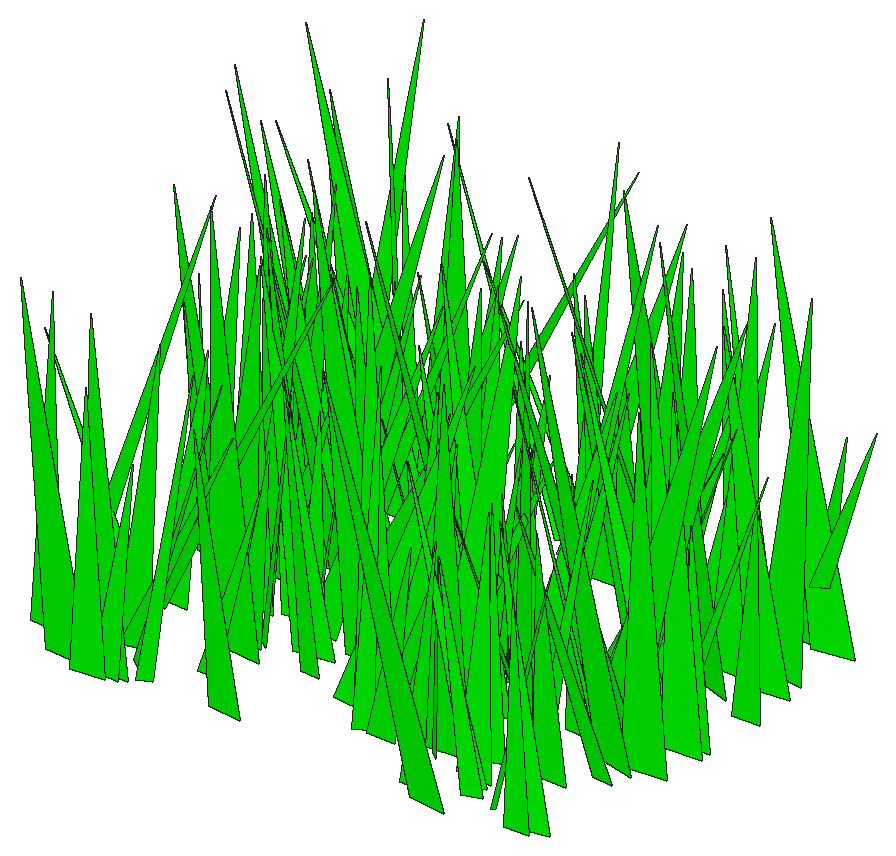
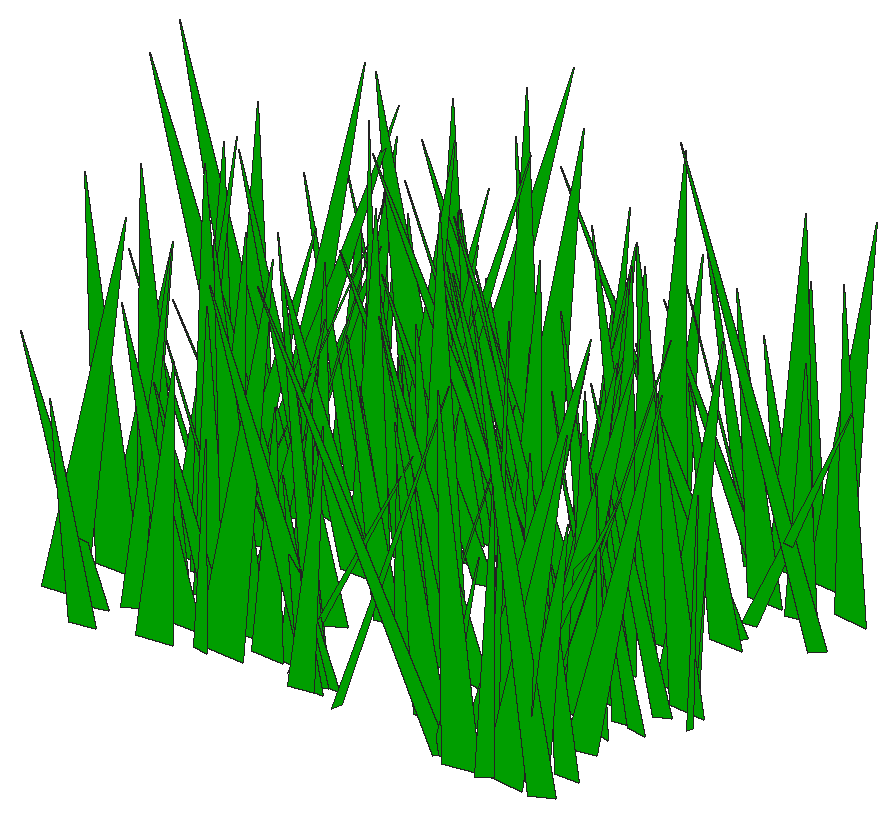
# SketchUp Ruby script. Lengths in inches.
U = 1.inch
M = Sketchup.active_model
def pt(a) = Geom::Point3d.new(a.map { |v| v * U })
def face(e, loops, mat)
  f = e.add_face(loops[0].map { |a| pt(a) })
  loops[1..].each { |l| e.add_face(l.map { |a| pt(a) }).erase! }
  f.material = f.back_material = mat if mat
  f
end
# faces: each face lists its corners as indices into pts; further lists are holes
def faces(e, pts, list, mat = nil) = list.each { |f| face(e, (f[0].is_a?(Array) ? f : [f]).map { |l| l.map { |i| pts[i] } }, mat) }
# xy, xz, yz: faces in a plane at the given z, y or x. An outline is a flat list of corners, or four numbers for a rectangle; further outlines are holes
def ring(l) = l.size == 4 ? [[l[0], l[1]], [l[2], l[1]], [l[2], l[3]], [l[0], l[3]]] : l.each_slice(2).to_a
def flat(e, list, mat, &to3) = list.each { |f| face(e, (f[0].is_a?(Array) ? f : [f]).map { |l| ring(l).map { |u, v| to3.(u, v) } }, mat) }
def xy(e, z, list, mat = nil) = flat(e, list, mat) { |x, y| [x, y, z] }
def xz(e, y, list, mat = nil) = flat(e, list, mat) { |x, z| [x, y, z] }
def yz(e, x, list, mat = nil) = flat(e, list, mat) { |y, z| [x, y, z] }
def lines(e, pts, list) = list.each { |a, b| e.add_line(pt(pts[a]), pt(pts[b])) }
# prism: a flat outline (further loops are holes) pulled along v
def prism(e, loops, v, mat = nil)
  f = face(e, loops, mat); d = Geom::Vector3d.new(v.map { |x| x * U })
  f.pushpull(f.normal.samedirection?(d) ? d.length : -d.length)
end
def box(e, o, s, mat = nil) = prism(e, [[o, [o[0] + s[0], o[1], o[2]], [o[0] + s[0], o[1] + s[1], o[2]], [o[0], o[1] + s[1], o[2]]]], [0, 0, s[2]], mat)
def at(x, y, z, deg = 0) = Geom::Transformation.translation(pt([x, y, z])) * Geom::Transformation.rotation(ORIGIN, Z_AXIS, deg.degrees)
def axes(o, x, y, z) = Geom::Transformation.new([*x, 0, *y, 0, *z, 0, *pt(o).to_a, 1])
def part(name) = M.definitions.add(name)
# library, detail: a bought-in or finely detailed component or shape, given as its bounding box
def library(name, o, s) = part(name).tap { |d| box(d.entities, o, s) }
def detail(e, o, s) = box(e.add_group.entities, o, s)
def put(e, d, t, mat = nil) = e.add_instance(d, t).tap { |i| i.material = mat if mat }
def group(e, t, mat = nil) = e.add_group.tap { |g| g.transformation = t; g.material = mat if mat }.entities
root = M.entities
M.materials.add("[0065_Lime]").color = [0, 255, 0]
c1 = part("fur_instance\#9")
p = [[0.8125,0,1.79],[0.67,-0.02,1.48],[0,-0.11,0],[0,0.11,0]]
faces(c1.entities,p,[[0,1,2,3]])
put(root,c1,axes([148.79,27.41,1.48],[-4.36413,0.0679,1.42951],[-0.40399,-0.66089,0.23585],[1.7773,0.0165,3.56374]),"[0065_Lime]")
put(root,c1,axes([150.34,30.25,1.48],[-6.51541,0.60637,1.27175],[-4.41577,-0.93218,-0.07461],[1.25175,-0.13226,6.35627]),"[0065_Lime]")
put(root,c1,axes([149.14,19.9,1.48],[3.62959,0.6982,2.01127],[-5.3272,0.55472,-0.09199],[-1.55669,-0.27041,5.00428]),"[0065_Lime]")
put(root,c1,axes([151.2,21.77,1.48],[-5.0487,0.24124,0.28222],[-1.73587,-0.70899,-0.23839],[0.23344,-0.05474,4.33106]),"[0065_Lime]")
put(root,c1,axes([150.35,32.46,1.48],[-2.61436,0.73575,0.51064],[-5.26778,-0.36894,-0.03169],[0.24537,-0.08138,4.76031]),"[0065_Lime]")
put(root,c1,axes([150.42,25.97,1.48],[-3.24186,-0.87839,1.38716],[6.44284,-0.46548,0.08559],[0.68891,0.21971,5.72721]),"[0065_Lime]")
put(root,c1,axes([152.13,32.04,1.48],[-6.23995,0.33949,0.21467],[-2.42526,-0.87643,-0.1994],[0.15736,-0.04553,5.43917]),"[0065_Lime]")
put(root,c1,axes([150.11,25.82,1.48],[-3.10048,-0.49021,1.16814],[3.63883,-0.45753,-0.04358],[0.99584,0.14559,3.79617]),"[0065_Lime]")
put(root,c1,axes([149.48,26.69,1.48],[2.5445,0.77902,1.23454],[-5.70579,0.37053,-0.05376],[-0.69495,-0.18982,4.96153]),"[0065_Lime]")
put(root,c1,axes([150.26,20.69,1.48],[-2.31714,0.67871,0.78015],[-4.863,-0.33882,0.32078],[0.77494,-0.09683,4.34572]),"[0065_Lime]")
put(root,c1,axes([150.95,32.95,1.48],[-3.51919,-0.90206,0.91897],[6.49484,-0.50053,-0.00735],[0.55111,0.13859,5.95488]),"[0065_Lime]")
put(root,c1,axes([150.71,18.86,1.48],[-2.47516,-0.99817,1.03588],[7.20412,-0.35294,-0.007],[0.42726,0.16858,6.11882]),"[0065_Lime]")
put(root,c1,axes([149.74,31.65,1.48],[2.54664,-0.49635,0.67652],[3.56798,0.36853,0.17373],[-0.66219,0.07682,3.53783]),"[0065_Lime]")
put(root,c1,axes([150.4,29.22,1.48],[4.29122,0.27494,1.64911],[-2.16036,0.65427,0.06434],[-1.80871,-0.12918,3.83571]),"[0065_Lime]")
put(root,c1,axes([150.35,28.31,1.48],[-0.84315,0.57058,1.0024],[-4.1932,-0.13912,0.31998],[0.65123,-0.15706,3.35818]),"[0065_Lime]")
put(root,c1,axes([152.72,28.54,1.48],[-8.21693,-0.01318,1.13181],[0.1147,-1.17091,0.0942],[1.38986,0.01873,6.68353]),"[0065_Lime]")
put(root,c1,axes([149.86,28.42,1.48],[4.47885,0.44067,1.13492],[-3.27298,0.6454,0.14884],[-1.03398,-0.13413,4.44494]),"[0065_Lime]")
put(root,c1,axes([149.6,32.9,1.48],[8.12572,-0.44878,2.16792],[3.45574,1.18577,-0.34466],[-2.31551,0.19477,7.09341]),"[0065_Lime]")
put(root,c1,axes([153.06,30.97,1.48],[-6.84359,0.82325,1.04818],[-5.93268,-0.96951,-0.11241],[0.888,-0.13265,7.32705]),"[0065_Lime]")
put(root,c1,axes([149.8,27.35,1.48],[5.49629,-0.3427,1.04891],[2.54858,0.78539,-0.23751],[-1.05618,0.11176,4.88535]),"[0065_Lime]")
put(root,c1,axes([152.9,28.39,1.48],[-5.44512,0.81928,0.57797],[-5.84746,-0.76896,0.07546],[0.55302,-0.06403,6.48869]),"[0065_Lime]")
put(root,c1,axes([148.77,21.8125,1.48],[8.96631,-0.27952,1.20894],[2.07914,1.27292,-0.34069],[-1.35758,0.10339,7.46286]),"[0065_Lime]")
put(root,c1,axes([151.53,33.01,1.48],[4.79868,-0.27542,2.30571],[2.45954,0.752,-0.37685],[-2.41398,0.2187,4.19947]),"[0065_Lime]")
put(root,c1,axes([150.98,23.09,1.48],[1.12346,0.7263,0.48945],[-5.2036,0.15631,0.13012],[0.02958,-0.08739,4.30055]),"[0065_Lime]")
put(root,c1,axes([151.43,28.74,1.48],[0.01172,-0.86138,1.50865],[6.40374,-0.00241,-0.0791],[0.09805,0.26061,4.98564]),"[0065_Lime]")
put(root,c1,axes([151.68,18.52,1.48],[2.09913,-0.70362,1.50752],[5.2611,0.3203,0.16253],[-0.91075,0.22854,4.41349]),"[0065_Lime]")
put(root,c1,axes([152.05,18.86,1.48],[-0.25767,-0.97075,1.60265],[7.18374,-0.03309,0.09255],[-0.04481,0.27725,5.62253]),"[0065_Lime]")
put(root,c1,axes([151.6,20.58,1.48],[-1.72483,-0.69834,2.52164],[5.7197,-0.29869,-0.18322],[1.26251,0.39911,4.27508]),"[0065_Lime]")
put(root,c1,axes([153.33,27.33,1.48],[-3.5745,0.80506,1.18789],[-5.8964,-0.50306,-0.31516],[0.43543,-0.2033,5.48383]),"[0065_Lime]")
put(root,c1,axes([152.51,25.98,1.48],[-4.00223,-0.90125,2.10909],[6.72796,-0.60506,-0.21665],[1.61068,0.28797,6.14564]),"[0065_Lime]")
put(root,c1,axes([151.72,27.625,1.48],[5.11006,0.68956,1.8792],[-5.18749,0.75159,0.09178],[-1.58391,-0.23686,5.76212]),"[0065_Lime]")
put(root,c1,axes([152.63,31.23,1.48],[-7.71879,0.02554,2.62939],[-0.23364,-1.17565,-0.07117],[3.2292,-0.02402,6.2799]),"[0065_Lime]")
put(root,c1,axes([152.12,18.74,1.48],[1.87428,-0.53121,1.16421],[4.03342,0.26043,-0.31441],[-0.2674,0.20491,3.41778]),"[0065_Lime]")
put(root,c1,axes([153.26,32.86,1.48],[-3.32693,-0.35067,0.66461],[2.48998,-0.48014,-0.24201],[0.83389,0.03463,3.37421]),"[0065_Lime]")
put(root,c1,axes([152.79,24.25,1.48],[-1.94674,1.02865,1.33122],[-7.46481,-0.28903,0.26114],[0.73764,-0.21018,6.15598]),"[0065_Lime]")
put(root,c1,axes([154.14,28.61,1.48],[-6.99031,0.25981,1.29728],[-1.87125,-1.00659,0.08387],[1.56868,-0.04296,5.88095]),"[0065_Lime]")
put(root,c1,axes([152.34,33.05,1.48],[-4.15139,0.72337,2.54398],[-5.55891,-0.66564,0.34035],[2.31965,-0.30058,5.36851]),"[0065_Lime]")
put(root,c1,axes([152.79,30.7,1.48],[-1.25112,0.54357,1.95893],[-4.51272,-0.19645,-0.08032],[0.63168,-0.32685,3.30604]),"[0065_Lime]")
put(root,c1,axes([151.82,26.96,1.48],[2.68129,-0.44256,0.1757],[3.15683,0.3761,-0.13073],[-0.01738,0.03775,3.36194]),"[0065_Lime]")
put(root,c1,axes([154.49,28.1875,1.48],[-3.65211,0.5727,0.51235],[-4.10393,-0.51635,-0.01487],[0.40664,-0.06764,4.45142]),"[0065_Lime]")
put(root,c1,axes([152.69,23.69,1.48],[1.95412,-1.01473,0.94427],[7.3129,0.27409,-0.14313],[-0.13127,0.16395,6.08353]),"[0065_Lime]")
put(root,c1,axes([151.42,29.86,1.48],[7.11093,-0.6367,0.78963],[4.53835,1.00737,0.17716],[-0.93622,0.0473,6.85629]),"[0065_Lime]")
put(root,c1,axes([151.57,20.45,1.48],[4.99654,-0.31795,0.05334],[2.26224,0.70216,0.03932],[-0.07968,-0.00239,4.4614]),"[0065_Lime]")
put(root,c1,axes([154.18,24.53,1.48],[-6.0982,0.47199,1.82636],[-3.42057,-0.90714,0.29884],[2.15021,-0.10449,5.65514]),"[0065_Lime]")
put(root,c1,axes([154.85,26.01,1.48],[-4.90548,-0.57351,0.82662],[4.11574,-0.69974,-0.10754],[0.86666,0.07685,5.18955]),"[0065_Lime]")
put(root,c1,axes([152.92,24.41,1.48],[5.49492,0.74794,1.88669],[-5.57567,0.80493,0.05163],[-1.6198,-0.23346,6.22259]),"[0065_Lime]")
put(root,c1,axes([154.09,21.99,1.48],[-3.45461,-1.10434,1.92252],[8.10797,-0.51503,-0.27371],[1.26988,0.28407,6.97767]),"[0065_Lime]")
put(root,c1,axes([152.37,19.8,1.48],[6.09642,0.17161,0.94555],[-1.28497,0.86964,0.19285],[-1.0916,-0.06529,5.05375]),"[0065_Lime]")
put(root,c1,axes([150.86,22.63,1.48],[8.41017,-0.22125,0.29815],[1.59286,1.18069,-0.3697],[-0.27606,0.0723,6.94997]),"[0065_Lime]")
put(root,c1,axes([153.17,19.19,1.48],[5.95695,-0.26908,1.45668],[1.98364,0.87102,0.02436],[-1.71442,0.07285,5.08961]),"[0065_Lime]")
put(root,c1,axes([154.07,22.57,1.48],[0.90778,-0.60694,0.27997],[4.32834,0.12473,-0.22464],[0.20044,0.05524,3.58308]),"[0065_Lime]")
put(root,c1,axes([154.8125,26.89,1.48],[-0.65002,0.54931,0.87031],[-4.04695,-0.09627,0.03628],[0.22106,-0.14724,3.22326]),"[0065_Lime]")
put(root,c1,axes([155.47,23.52,1.48],[4.82868,0.68716,3.43263],[-5.75973,0.79317,0.04022],[-2.9237,-0.42767,5.58997]),"[0065_Lime]")
put(root,c1,axes([155.96,23.16,1.48],[-4.17571,0.84117,1.42735],[-6.19547,-0.59384,-0.26526],[0.72784,-0.229,5.93093]),"[0065_Lime]")
put(root,c1,axes([154.4375,22.86,1.48],[4.74754,0.15255,1.39795],[-1.26444,0.70201,0.27418],[-1.59168,-0.10267,3.95189]),"[0065_Lime]")
put(root,c1,axes([154.98,24.26,1.48],[0.48111,0.61612,0.39007],[-4.40537,0.07047,-0.13493],[-0.21813,-0.06438,3.58537]),"[0065_Lime]")
put(root,c1,axes([154.64,31.5,1.48],[2.09332,0.7765,0.81963],[-5.60135,0.29988,-0.05449],[-0.42048,-0.12902,4.80631]),"[0065_Lime]")
put(root,c1,axes([157.16,32.48,1.48],[-7.47411,0.1121,0.86388],[-0.74162,-1.05975,0.36283],[1.10199,0.04713,6.1033]),"[0065_Lime]")
put(root,c1,axes([154.27,20.56,1.48],[3.19346,-0.36854,0.66312],[2.7234,0.44766,-0.34073],[-0.35576,0.11869,3.34407]),"[0065_Lime]")
put(root,c1,axes([156.01,19.15,1.48],[-2.25642,-0.73712,0.7058],[5.28021,-0.32622,-0.2473],[0.62486,0.09477,4.63839]),"[0065_Lime]")
put(root,c1,axes([154.45,25.95,1.48],[5.61294,0.61264,0.91241],[-4.38547,0.80101,-0.17237],[-1.01707,-0.07284,5.7786]),"[0065_Lime]")
put(root,c1,axes([155.22,24.05,1.48],[3.95693,-0.03593,0.88991],[0.14238,0.57433,0.35811],[-1.11447,-0.05419,3.20539]),"[0065_Lime]")
put(root,c1,axes([156.5,22.3,1.48],[-4.27742,-0.44205,1.63992],[3.45962,-0.63123,0.26888],[1.4115,0.20755,4.31061]),"[0065_Lime]")
put(root,c1,axes([156.47,25.12,1.48],[-2.90347,-0.86262,1.44057],[6.28485,-0.43481,-0.34361],[1.15038,0.1983,5.51311]),"[0065_Lime]")
put(root,c1,axes([154.92,29.2,1.48],[4.25717,0.85419,0.2085],[-6.07405,0.59922,-0.20402],[-0.35253,-0.00926,6.03316]),"[0065_Lime]")
put(root,c1,axes([156.3,28.93,1.48],[3.11019,-1.09853,2.30406],[8.21919,0.47052,0.17634],[-1.25928,0.35783,6.84156]),"[0065_Lime]")
put(root,c1,axes([153.21,32.81,1.48],[8.28377,-0.25525,0.1321],[1.82152,1.16322,-0.25907],[-0.09028,0.04861,6.89336]),"[0065_Lime]")
put(root,c1,axes([157.51,23.85,1.48],[-2.45409,-1.24152,1.7361],[9.08856,-0.33956,0.36348],[0.12847,0.30588,7.44999]),"[0065_Lime]")
put(root,c1,axes([154.54,26.16,1.48],[7.83343,0.51256,0.68917],[-3.66744,1.10586,0.02138],[-0.75691,-0.05362,7.02871]),"[0065_Lime]")
put(root,c1,axes([159.34,31.71,1.48],[-5.63037,0.09906,0.11334],[-0.70447,-0.79141,0.0225],[0.1417,0.00143,4.61551]),"[0065_Lime]")
put(root,c1,axes([155.27,24.33,1.48],[5.55044,0.73634,0.39249],[-5.25052,0.78151,-0.0023],[-0.3528,-0.04626,6.20901]),"[0065_Lime]")
put(root,c1,axes([156.73,28.67,1.48],[0.7258,-0.88641,0.96905],[6.41504,0.09375,-0.30543],[0.24361,0.17215,5.15595]),"[0065_Lime]")
put(root,c1,axes([157.375,28.83,1.48],[-1.16934,0.86799,0.44277],[-6.17523,-0.17009,0.38303],[0.56537,-0.06259,5.09942]),"[0065_Lime]")
put(root,c1,axes([158.73,25.41,1.48],[-4.26167,-0.00508,0.56307],[0.06727,-0.60606,0.15354],[0.68991,0.0277,3.46322]),"[0065_Lime]")
put(root,c1,axes([158.56,32.31,1.48],[3.46598,-0.43735,2.28282],[3.64792,0.56676,-0.02608],[-2.06306,0.26739,3.78908]),"[0065_Lime]")
put(root,c1,axes([158.49,22.36,1.48],[-0.97898,0.63149,0.10351],[-4.49076,-0.13822,0.15503],[0.21336,-0.01175,3.73801]),"[0065_Lime]")
put(root,c1,axes([158.33,31.75,1.48],[3.34876,-0.35125,1.19294],[2.65277,0.49831,-0.01051],[-1.16707,0.12481,3.39909]),"[0065_Lime]")
put(root,c1,axes([155.46,25.25,1.48],[7.99127,-0.42176,0.12754],[3.0053,1.12214,-0.24314],[-0.04157,0.04707,6.93932]),"[0065_Lime]")
put(root,c1,axes([158.29,32.22,1.48],[2.2006,-0.49727,0.10109],[3.53061,0.3097,0.19686],[-0.27113,-0.00316,3.38397]),"[0065_Lime]")
put(root,c1,axes([158.26,31.91,1.48],[7.84742,-0.32487,2.282],[2.41765,1.16677,0.06512],[-2.7149,0.09999,6.65413]),"[0065_Lime]")
put(root,c1,axes([159.47,31.4375,1.48],[1.07815,0.70024,1.60621],[-5.28991,0.18471,-0.34901],[-0.8658,-0.25657,4.13257]),"[0065_Lime]")
put(root,c1,axes([161.25,24.26,1.48],[-7.70626,-0.58047,1.23862],[4.24714,-1.09378,0.30701],[1.15983,0.14844,7.10555]),"[0065_Lime]")
put(root,c1,axes([158.75,26.45,1.48],[1.68717,-0.5842,1.18376],[4.40076,0.23298,-0.29712],[-0.1896,0.20915,3.6375]),"[0065_Lime]")
put(root,c1,axes([158.32,23.49,1.48],[4.05903,0.53982,1.0784],[-4.00493,0.57606,0.31103],[-0.69049,-0.16786,4.53532]),"[0065_Lime]")
put(root,c1,axes([159.55,21.41,1.48],[5.33526,-0.81935,2.96567],[6.39191,0.83004,0.07602],[-2.53698,0.36819,6.42833]),"[0065_Lime]")
put(root,c1,axes([159.02,27.92,1.48],[-2.63979,0.50784,2.41439],[-4.19679,-0.46858,0.26665],[2.06369,-0.3033,3.63065]),"[0065_Lime]")
put(root,c1,axes([159.29,27.36,1.48],[3.84746,0.1933,0.97119],[-1.42879,0.56346,-0.01291],[-1.12983,-0.0543,3.32357]),"[0065_Lime]")
put(root,c1,axes([159.55,20.82,1.48],[-6.10363,0.31379,2.82473],[-2.64016,-0.96623,-0.17783],[3.17426,-0.20028,5.28364]),"[0065_Lime]")
put(root,c1,axes([161.11,23.71,1.48],[-4.12674,0.75773,0.57064],[-5.40533,-0.58511,0.17075],[0.59374,-0.06023,5.52066]),"[0065_Lime]")
put(root,c1,axes([158.28,31.76,1.48],[4.58827,0.88238,0.39675],[-6.29659,0.64466,0.13585],[-0.15257,-0.0692,6.32461]),"[0065_Lime]")
put(root,c1,axes([158.24,24.62,1.48],[4.74852,-0.43104,0.1658],[3.07422,0.66614,-0.22345],[-0.02185,0.04797,4.59292]),"[0065_Lime]")
put(root,c1,axes([159.71,22.79,1.48],[3.79608,-0.64754,1.81741],[4.98008,0.55789,-0.22168],[-1.19451,0.26807,4.85137]),"[0065_Lime]")
put(root,c1,axes([158.49,21.69,1.48],[4.67576,0.91116,0.07172],[-6.48482,0.65704,0.01908],[-0.03254,-0.01198,6.50265]),"[0065_Lime]")
put(root,c1,axes([160.4,31.5,1.48],[1.25266,-0.66556,0.7393],[4.78923,0.18723,0.27893],[-0.56899,0.11064,3.97541]),"[0065_Lime]")
put(root,c1,axes([160.11,23.04,1.48],[2.223,-0.6266,1.62727],[4.86649,0.31234,-0.36854],[-0.45189,0.28115,4.03614]),"[0065_Lime]")
put(root,c1,axes([161.81,23.74,1.48],[-6.69213,0.67949,1.58645],[-4.87096,-0.9738,0.3812],[1.86033,-0.10541,6.70501]),"[0065_Lime]")
put(root,c1,axes([161.55,32.12,1.48],[-3.07955,-1.06505,0.8199],[7.61697,-0.44065,-0.25151],[0.66777,0.11465,6.64993]),"[0065_Lime]")
put(root,c1,axes([160.23,20.76,1.48],[1.45682,-0.5883,0.2555],[4.1972,0.20294,-0.1762],[0.10199,0.05167,3.60146]),"[0065_Lime]")
put(root,c1,axes([159.64,21.87,1.48],[3.91301,-0.43156,0.02337],[3.06066,0.54846,0.30755],[-0.25598,-0.03931,4.03448]),"[0065_Lime]")
put(root,c1,axes([163.78,29.7,1.48],[-8.56016,-0.07019,0.67398],[0.53969,-1.20684,0.32355],[0.803,0.06283,6.96728]),"[0065_Lime]")
put(root,c1,axes([160.7,24.87,1.48],[2.71996,-0.63123,0.39601],[4.50795,0.38454,0.05327],[-0.3084,0.05373,4.27128]),"[0065_Lime]")
put(root,c1,axes([161.61,25.49,1.48],[2.92369,-0.83085,1.74803],[6.14317,0.44884,0.35047],[-1.35671,0.24189,5.35392]),"[0065_Lime]")
put(root,c1,axes([162.62,29.01,1.48],[-4.29958,-0.57338,0.94433],[4.1671,-0.61436,0.05366],[0.79576,0.11914,4.8213]),"[0065_Lime]")
put(root,c1,axes([159.8125,23.92,1.48],[4.38526,0.5456,0.02818],[-3.88076,0.6156,0.19029],[0.12917,-0.02784,4.76049]),"[0065_Lime]")
put(root,c1,axes([160,28.96,1.48],[8.11748,-0.39096,1.56123],[2.90393,1.16571,-0.20812],[-1.72984,0.12226,6.97685]),"[0065_Lime]")
put(root,c1,axes([161.21,23.96,1.48],[4.06678,0.47502,0.9917],[-3.40207,0.59225,-0.27538],[-1.15773,-0.07175,4.29279]),"[0065_Lime]")
put(root,c1,axes([163.59,18.59,1.48],[-5.69989,-0.84067,0.92357],[6.04407,-0.80766,0.04546],[0.74235,0.12098,6.72129]),"[0065_Lime]")
put(root,c1,axes([160.82,28.28,1.48],[4.97241,-0.33385,0.80836],[2.38692,0.71144,0.13126],[-0.967,0.03939,4.48069]),"[0065_Lime]")
put(root,c1,axes([161.13,23,1.48],[1.90323,1.25548,1.09793],[-9.03556,0.26234,0.31094],[0.09697,-0.19666,7.42415]),"[0065_Lime]")
put(root,c1,axes([162.09,32.33,1.48],[-3.15964,-0.31029,1.33421],[2.40714,-0.48178,0.01716],[1.33131,0.13467,3.1355]),"[0065_Lime]")
put(root,c1,axes([162,20.9,1.48],[-4.79954,-0.15707,1.8677],[1.07368,-0.74733,-0.28042],[2.31707,0.02095,3.99866]),"[0065_Lime]")
put(root,c1,axes([161.64,30.92,1.48],[2.89516,-0.93665,1.66085],[6.94732,0.41346,-0.19939],[-0.57942,0.27727,5.90796]),"[0065_Lime]")
put(root,c1,axes([162.14,21.2,1.48],[1.76652,-1.06791,0.87729],[7.65641,0.25623,0.25084],[-0.54722,0.1376,6.34162]),"[0065_Lime]")
put(root,c1,axes([161.3,26.34,1.48],[2.10443,0.84787,0.02122],[-6.02631,0.29514,0.269],[0.30368,-0.01876,5.19103]),"[0065_Lime]")
put(root,c1,axes([162.5,24.16,1.48],[-6.55122,-0.45777,2.93134],[3.80766,-1.01182,0.33559],[3.0169,0.28298,5.94188]),"[0065_Lime]")
put(root,c1,axes([164.07,20.18,1.48],[-5.3336,0.35172,1.04866],[-2.61898,-0.76221,-0.2469],[1.03353,-0.11638,4.78604]),"[0065_Lime]")
put(root,c1,axes([161.72,31.76,1.48],[2.97008,0.56166,0.51449],[-4.04561,0.41481,0.27826],[-0.09957,-0.10007,4.04105]),"[0065_Lime]")
put(root,c1,axes([163.42,32.68,1.48],[-2.52787,0.7902,0.5342],[-5.63626,-0.36079,0.23678],[0.53597,-0.06721,5.00951]),"[0065_Lime]")
put(root,c1,axes([162.57,19.18,1.48],[2.86367,0.55216,0.94086],[-3.98635,0.42128,-0.25682],[-0.94209,-0.10422,3.94665]),"[0065_Lime]")
put(root,c1,axes([164.94,22.03,1.48],[-4.38503,-0.23062,0.34414],[1.67767,-0.61406,0.35456],[0.2411,0.07835,3.79195]),"[0065_Lime]")
put(root,c1,axes([163.83,22.39,1.48],[-3.99106,-0.32596,1.5368],[2.62685,-0.59364,0.29439],[1.43191,0.18051,3.74336]),"[0065_Lime]")
put(root,c1,axes([163.61,21.64,1.48],[4.1483,-0.2647,1.80841],[2.12462,0.64671,-0.05273],[-1.99427,0.13838,3.7055]),"[0065_Lime]")
put(root,c1,axes([164.25,19.74,1.48],[-3.16464,0.40378,1.16817],[-3.11583,-0.45476,-0.31766],[0.78183,-0.17795,3.46247]),"[0065_Lime]")
put(root,c1,axes([163.63,20.59,1.48],[-0.45419,0.75663,0.45252],[-5.40529,-0.06765,0.20072],[0.2939,-0.07488,4.39089]),"[0065_Lime]")
put(root,c1,axes([163.62,29.97,1.48],[2.26816,-0.6951,1.41808],[5.17158,0.34087,0.12588],[-0.87405,0.21307,4.42474]),"[0065_Lime]")
put(root,c1,axes([165.36,23.97,1.48],[-6.56763,-0.02491,1.05288],[0.13962,-0.94029,-0.16917],[1.299,-0.02487,5.34147]),"[0065_Lime]")
put(root,c1,axes([163.63,28.92,1.48],[1.48957,-0.59927,0.62365],[4.32036,0.21413,0.06726],[-0.33196,0.09781,3.67388]),"[0065_Lime]")
put(root,c1,axes([164.27,24.31,1.48],[-3.26223,-0.44125,1.79337],[3.58749,-0.49499,0.23676],[1.36063,0.24718,3.6755]),"[0065_Lime]")
put(root,c1,axes([163.27,31.59,1.48],[1.94891,0.85485,0.64198],[-6.13363,0.26949,0.29514],[0.10778,-0.12112,5.18781]),"[0065_Lime]")
put(root,c1,axes([165.76,26.15,1.48],[-5.77336,0.49165,0.80714],[-3.51927,-0.82122,0.10662],[0.91712,-0.05633,5.49016]),"[0065_Lime]")
put(root,c1,axes([165.06,31.64,1.48],[-6.68438,0.34926,1.83375],[-2.5314,-0.98834,0.20247],[2.20274,-0.07596,5.79734]),"[0065_Lime]")
put(root,c1,axes([162.35,28.03,1.48],[5.19294,0.17912,0.05057],[-1.26712,0.72799,-0.31418],[-0.15231,0.05064,4.33804]),"[0065_Lime]")
put(root,c1,axes([166.51,23.91,1.48],[-7.03028,-0.71093,0.82217],[5.10266,-0.99358,0.07982],[0.76264,0.09423,7.04494]),"[0065_Lime]")
put(root,c1,axes([164.8,27.8,1.48],[-4.02525,0.6943,1.64967],[-5.16684,-0.59658,0.07208],[1.35291,-0.21267,5.18345]),"[0065_Lime]")
put(root,c1,axes([162.9375,29.38,1.48],[5.09244,0.01356,0.56709],[-0.06815,0.7217,-0.17321],[-0.70051,0.02834,4.13938]),"[0065_Lime]")
put(root,c1,axes([164.28,28.97,1.48],[-3.12736,0.88903,3.18912],[-7.2505,-0.49895,-0.04344],[1.68251,-0.49767,5.74056]),"[0065_Lime]")
put(root,c1,axes([165.875,28.46,1.48],[-7.31235,-0.55627,1.97575],[4.02465,-1.07665,-0.30212],[2.31811,0.11452,6.75692]),"[0065_Lime]")
put(root,c1,axes([166.26,23.47,1.48],[-6.31931,-0.8589,1.30862],[6.14598,-0.90962,-0.36892],[1.47538,0.11039,7.14182]),"[0065_Lime]")
put(root,c1,axes([166.49,22.68,1.48],[-3.85506,-0.48643,0.32778],[3.48051,-0.54169,0.14723],[0.17835,0.05679,4.21189]),"[0065_Lime]")
put(root,c1,axes([164.35,22.7,1.48],[5.39035,-0.2698,1.27807],[2.03158,0.78311,-0.12956],[-1.42414,0.09592,4.65264]),"[0065_Lime]")
put(root,c1,axes([165.375,21.74,1.48],[-0.19329,-0.73306,0.46325],[5.24759,-0.02774,-0.02251],[0.04891,0.07983,4.24629]),"[0065_Lime]")
put(root,c1,axes([165.61,29.58,1.48],[0.12495,1.15956,1.24234],[-8.39122,0.01396,0.12181],[0.12916,-0.21488,6.712]),"[0065_Lime]")
put(root,c1,axes([167.03,32.16,1.48],[-5.09611,0.86284,1.48409],[-6.33271,-0.72795,-0.20586],[0.96484,-0.22048,6.48753]),"[0065_Lime]")
put(root,c1,axes([166.33,27.25,1.48],[-3.95863,0.06757,1.15622],[-0.42218,-0.5909,0.20085],[1.43998,0.01253,3.23745]),"[0065_Lime]")
put(root,c1,axes([167.04,29.34,1.48],[-2.45359,0.90234,0.89479],[-6.51502,-0.34052,-0.31342],[0.02749,-0.16374,5.58287]),"[0065_Lime]")
put(root,c1,axes([165.125,19.6,1.48],[4.96286,-0.02698,0.95466],[0.26641,0.71494,-0.23931],[-1.15902,0.04881,4.03278]),"[0065_Lime]")
put(root,c1,axes([165.5,33.28,1.48],[1.09423,-0.58718,0.26778],[4.18087,0.14946,-0.32157],[0.3005,0.05868,3.49887]),"[0065_Lime]")
put(root,c1,axes([166.92,19.25,1.48],[-4.37945,0.49598,1.3584],[-3.7105,-0.63843,-0.10383],[1.21636,-0.16179,4.57408]),"[0065_Lime]")
put(root,c1,axes([166.42,18.99,1.48],[1.33705,0.58663,1.07878],[-4.31493,0.20994,-0.28707],[-0.75435,-0.1611,3.55415]),"[0065_Lime]")
put(root,c1,axes([163.97,26.65,1.48],[6.41409,-0.91946,0.4883],[6.56843,0.90039,-0.27493],[-0.17805,0.09352,7.44803]),"[0065_Lime]")
put(root,c1,axes([167.23,25.23,1.48],[-2.99848,0.80558,2.25489],[-6.25693,-0.45277,-0.08469],[1.18423,-0.3525,5.2619]),"[0065_Lime]")
put(root,c1,axes([165.08,25,1.48],[5.98232,-0.979,0.64405],[6.99921,0.84254,-0.09969],[-0.42244,0.09566,7.46895]),"[0065_Lime]")
put(root,c1,axes([167.11,23.74,1.48],[1.60834,-0.97379,1.48435],[7.13509,0.24208,0.20657],[-0.66767,0.2413,5.78311]),"[0065_Lime]")
put(root,c1,axes([166.62,30.27,1.48],[1.98996,0.97599,2.17109],[-7.43499,0.27622,0.34802],[-0.29536,-0.37757,5.86668]),"[0065_Lime]")
put(root,c1,axes([165.76,27.1,1.48],[4.96309,0.29977,0.47017],[-2.10141,0.70186,-0.31823],[-0.68502,0.0188,4.38265]),"[0065_Lime]")
put(root,c1,axes([167.42,25.67,1.48],[-0.6638,0.60158,0.56385],[-4.3365,-0.09341,-0.03819],[0.05922,-0.09727,3.52375]),"[0065_Lime]")
put(root,c1,axes([165.8,32.26,1.48],[3.70352,-0.48466,0.34357],[3.47421,0.51812,-0.28747],[-0.06664,0.07682,4.10651]),"[0065_Lime]")
put(root,c1,axes([167.47,27.79,1.48],[1.40347,-0.59563,0.86044],[4.35669,0.20244,-0.00581],[-0.32552,0.14143,3.632]),"[0065_Lime]")
